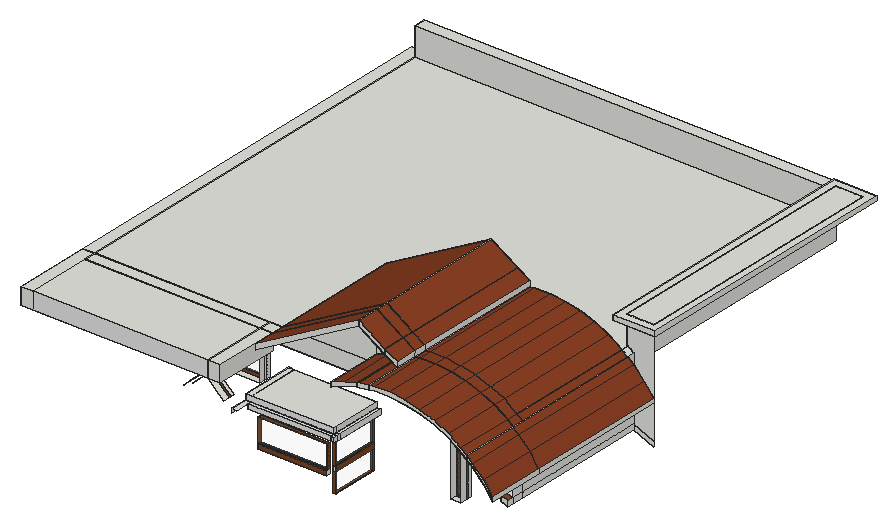
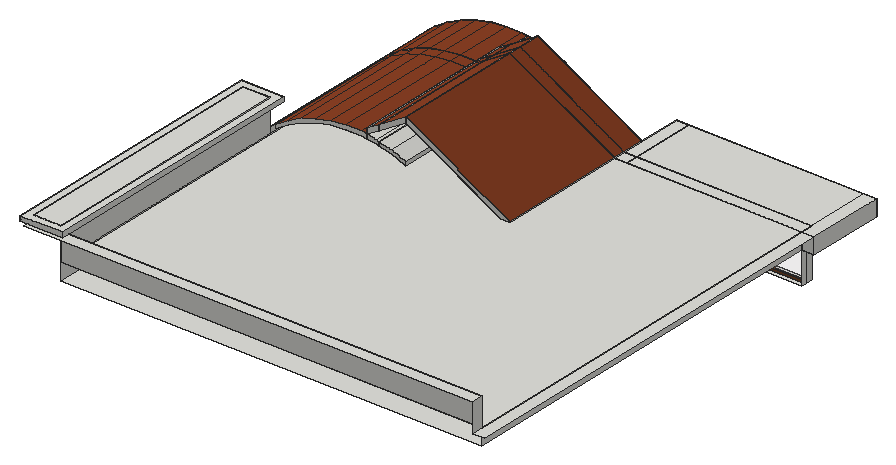
# SketchUp Ruby script. Lengths in inches.
U = 1.inch
M = Sketchup.active_model
def pt(a) = Geom::Point3d.new(a.map { |v| v * U })
def face(e, loops, mat)
  f = e.add_face(loops[0].map { |a| pt(a) })
  loops[1..].each { |l| e.add_face(l.map { |a| pt(a) }).erase! }
  f.material = f.back_material = mat if mat
  f
end
# faces: each face lists its corners as indices into pts; further lists are holes
def faces(e, pts, list, mat = nil) = list.each { |f| face(e, (f[0].is_a?(Array) ? f : [f]).map { |l| l.map { |i| pts[i] } }, mat) }
# xy, xz, yz: faces in a plane at the given z, y or x. An outline is a flat list of corners, or four numbers for a rectangle; further outlines are holes
def ring(l) = l.size == 4 ? [[l[0], l[1]], [l[2], l[1]], [l[2], l[3]], [l[0], l[3]]] : l.each_slice(2).to_a
def flat(e, list, mat, &to3) = list.each { |f| face(e, (f[0].is_a?(Array) ? f : [f]).map { |l| ring(l).map { |u, v| to3.(u, v) } }, mat) }
def xy(e, z, list, mat = nil) = flat(e, list, mat) { |x, y| [x, y, z] }
def xz(e, y, list, mat = nil) = flat(e, list, mat) { |x, z| [x, y, z] }
def yz(e, x, list, mat = nil) = flat(e, list, mat) { |y, z| [x, y, z] }
def lines(e, pts, list) = list.each { |a, b| e.add_line(pt(pts[a]), pt(pts[b])) }
# prism: a flat outline (further loops are holes) pulled along v
def prism(e, loops, v, mat = nil)
  f = face(e, loops, mat); d = Geom::Vector3d.new(v.map { |x| x * U })
  f.pushpull(f.normal.samedirection?(d) ? d.length : -d.length)
end
def box(e, o, s, mat = nil) = prism(e, [[o, [o[0] + s[0], o[1], o[2]], [o[0] + s[0], o[1] + s[1], o[2]], [o[0], o[1] + s[1], o[2]]]], [0, 0, s[2]], mat)
def at(x, y, z, deg = 0) = Geom::Transformation.translation(pt([x, y, z])) * Geom::Transformation.rotation(ORIGIN, Z_AXIS, deg.degrees)
def axes(o, x, y, z) = Geom::Transformation.new([*x, 0, *y, 0, *z, 0, *pt(o).to_a, 1])
def part(name) = M.definitions.add(name)
# library, detail: a bought-in or finely detailed component or shape, given as its bounding box
def library(name, o, s) = part(name).tap { |d| box(d.entities, o, s) }
def detail(e, o, s) = box(e.add_group.entities, o, s)
def put(e, d, t, mat = nil) = e.add_instance(d, t).tap { |i| i.material = mat if mat }
def group(e, t, mat = nil) = e.add_group.tap { |g| g.transformation = t; g.material = mat if mat }.entities
root = M.entities
M.materials.add("Glass Thin Clear 001").color = [243, 240, 240]
M.materials["Glass Thin Clear 001"].alpha = 0.1
M.materials.add("[Color M01]").color = [226, 226, 226]
M.materials.add("[Roofing Tile Spanish]").color = [138, 64, 36]
M.materials.add("[Wood Veneer 01]").color = [120, 70, 37]
xy(root,188.71,[[288.03,166.0625,295.34,170.5625],[288.03,170.5625,295.34,172.4375],[288.03,172.4375,295.34,172.5],[288.03,172.5,295.34,175.0625]])
xy(root,189.01,[[231.27,128.93,233.15,163.51],[233.15,128.93,233.59,163.51]],"[Wood Veneer 01]")
xy(root,189.7,[[289.02,170.5625,294.34,171.125],[289.02,171.125,294.34,172.5]],"[Wood Veneer 01]")
xy(root,200.48,[[177.78,126.375,228.77,127],[177.78,127,228.77,128.9375]],"[Wood Veneer 01]")
xy(root,203.62,[[231.27,128.93,233.15,163.51],[233.15,128.93,233.59,163.51]],"[Wood Veneer 01]")
xy(root,203.86,[[177.78,126.375,228.77,127],[177.78,127,228.77,128.9375]],"[Wood Veneer 01]")
xy(root,207.19,[[231.27,128.93,233.15,163.51],[233.15,128.93,233.59,163.51]],"[Wood Veneer 01]")
xy(root,216.17,[[18.96,166.0625,147.96,170.5625],[18.96,171.875,147.96,175.0625]])
xy(root,216.17,[[18.96,170.5625,147.96,171.5625],[18.96,171.5625,147.96,171.875]],"[Wood Veneer 01]")
xy(root,217.66,[[42.44,170.5625,44.71,171.875],[66.82,170.5625,69.08,171.875],[89.69,170.5625,91.96,171.875],[117,170.5625,119.27,171.875]])
xy(root,217.66,[[20.45,170.5625,42.44,170.875],[44.71,170.5625,66.82,170.875],[69.08,170.5625,89.69,170.875],[91.96,170.5625,117,170.875],[119.27,170.5625,146.47,170.875],
  [20.45,170.875,42.44,171.875],[44.71,170.875,66.82,171.875],[69.08,170.875,89.69,171.875],[91.96,170.875,117,171.875],[119.27,170.875,146.47,171.875]],"[Wood Veneer 01]")
xy(root,221.31,[[177.78,126.375,228.77,127],[177.78,127,228.77,128.9375]],"[Wood Veneer 01]")
xy(root,223.57,[[231.27,128.93,233.15,163.51],[233.15,128.93,233.59,163.51]],"[Wood Veneer 01]")
xy(root,226.125,[[172.96,123.625,233.59,126.375],[233.59,123.625,236.34,126.375],[168.96,126.375,172.96,166.0625],[172.96,126.375,231.27,128.3125],[233.59,126.375,236.34,128.5625],
  [172.96,128.3125,231.27,128.5625],[172.96,128.5625,231.27,128.9375],[233.59,128.5625,236.34,166.0625],[172.96,128.9375,231.27,166.0625],[231.34,128.9375,231.84,166.0625]])
xy(root,226.125,[[231.27,126.375,231.84,128.3125],[231.84,126.375,233.59,128.3125],[231.27,128.3125,231.84,128.5625],[231.84,128.3125,233.59,128.5625],[231.27,128.5625,231.34,128.9375],
  [231.34,128.5625,231.84,128.9375],[231.84,128.5625,233.59,128.9375],[231.27,128.9375,231.34,166.0625],[231.84,128.9375,233.59,166.0625]],"[Wood Veneer 01]")
xy(root,229.5625,[[168.96,113.5625,172.96,126.375],[172.96,123.625,233.59,126.375],[233.59,123.625,236.34,126.375],[168.96,126.375,172.96,166.0625],[172.96,126.375,233.59,128.5625],
  [233.59,126.375,236.34,128.5625],[172.96,128.5625,173.02,166.0625],[173.02,128.5625,233.59,166.0625],[233.59,128.5625,236.34,166.0625]])
xy(root,233.5,[[168.96,126.375,233.59,126.375,233.59,166.0625,173.02,166.0625,173.02,128.5625,172.96,128.5625,172.96,166.0625,168.96,166.0625],[172.96,128.5625,173.02,166.0625]])
xy(root,238.51,[[20.45,170.5625,42.44,170.875],[42.44,170.5625,44.71,171.875],[66.82,170.5625,69.08,171.875],[89.69,170.5625,91.96,171.875],[117,170.5625,119.27,171.875],
  [119.27,170.875,146.47,171.875]])
xy(root,238.51,[[44.71,170.5625,66.82,170.875],[69.08,170.5625,89.69,170.875],[91.96,170.5625,117,170.875],[119.27,170.5625,146.47,170.875],[20.45,170.875,42.44,171.875],
  [44.71,170.875,66.82,171.875],[69.08,170.875,89.69,171.875],[91.96,170.875,117,171.875]],"[Wood Veneer 01]")
xy(root,240,[[9.96,118.0625,18.96,166.0625],[18.96,118.0625,147.96,166.0625],[147.96,118.0625,156.96,166.0625],[9.96,166.0625,18.96,175.0625],[18.96,175.0625,328.85,469.0625]])
xy(root,240,[[18.96,170.5625,147.96,171.5625],[18.96,171.5625,147.96,171.875]],"[Wood Veneer 01]")
xy(root,252,[[9.96,118.0625,18.96,175.0625],[18.96,118.0625,147.96,166.0625],[147.96,118.0625,156.96,166.0625],[18.96,166.0625,147.96,175.0625],[147.96,166.0625,156.96,175.0625],
  [9.96,175.0625,18.96,478.0625],[18.96,175.0625,328.85,469.0625]])
xy(root,258.59,[[289.02,170.5625,294.34,171.125],[289.02,171.125,294.34,172.5]],"[Wood Veneer 01]")
xy(root,259.58,[[288.03,166.0625,295.34,170.5625],[288.03,172.5,295.34,175.0625]])
xy(root,259.58,[[288.03,170.5625,295.34,172.4375],[288.03,172.4375,295.34,172.5]],"[Wood Veneer 01]")
xy(root,259.6875,[[274.03,170.5625,280.57,171.125],[274.03,171.125,280.57,172.5]],"[Wood Veneer 01]")
xy(root,259.97,[[259.4375,170.5625,266.9,171.125],[259.4375,171.125,266.9,172.5]],"[Wood Veneer 01]")
xy(root,260.53,[[244.43,170.5625,251.95,170.8125],[244.43,170.8125,251.95,172.5]],"[Wood Veneer 01]")
xy(root,260.67,[[273.05,166.0625,281.55,170.5625],[273.05,172.5,281.55,175.0625]])
xy(root,260.67,[[273.05,170.5625,281.55,172.4375],[273.05,172.4375,281.55,172.5]],"[Wood Veneer 01]")
xy(root,261.18,[[258.23,166.0625,268.1,170.5625],[258.23,172.5,268.1,175.0625]])
xy(root,261.18,[[258.23,170.5625,268.1,172.4375],[258.23,172.4375,268.1,172.5]],"[Wood Veneer 01]")
xy(root,261.4,[[243.5625,166.0625,252.8125,170.5625],[243.5625,172.5,252.8125,175.0625]])
xy(root,261.4,[[243.5625,170.5625,252.8125,172.125],[243.5625,172.125,252.8125,172.5]],"[Wood Veneer 01]")
xy(root,272.68,[[323.41,271.25,323.41,469.0625,328.85,469.0625,328.85,276.6875,348.92,276.6875,348.92,474.5,354.36,474.5,354.36,271.25],[328.85,276.6875,348.92,469.0625],[18.96,469.0625,323.41,469.0625,323.41,474.5,348.92,474.5,348.92,478.0625,18.96,478.0625],[323.41,469.0625,348.92,474.5]])
xy(root,276.24,[[[323.41,271.25,354.36,474.5],[328.85,276.6875,348.92,469.0625]],[328.85,276.6875,348.92,469.0625]])
xz(root,118.0625,[[9.96,240,18.96,252],[147.96,240,156.96,252]])
xz(root,118.0625,[[18.96,240,147.96,252]],"[Color M01]")
xz(root,123.625,[[233.59,226.125,236.34,229.5625],[353.03,228.22,353.03,231.22,346.26,240.23,338.49,248.37,333.96,252.11,333.96,249.1,338.49,245.37,346.26,237.22],[333.96,249.1,333.96,252.11,329.8,255.54,320.33,261.63,310.2,266.5625,299.57,270.26,288.57,272.68,277.36,273.78,266.11,273.55,261.96,272.98,261.96,269.97,266.11,270.55,277.36,270.78,288.57,269.67,299.57,267.25,310.2,263.55,320.33,258.625,329.8,252.53],[233.59,262,244.0625,266.13,252.96,268.47,252.96,271.47,244.0625,269.14,233.59,265.01],[252.96,268.47,254.95,268.99,261.96,269.97,261.96,272.98,254.95,272,252.96,271.47]])
xz(root,123.625,[[172.96,226.125,233.59,229.5625]],"[Color M01]")
xz(root,126.375,[[168.96,226.125,172.96,229.5625],[172.96,226.125,233.59,229.5625],[233.59,226.125,236.34,229.5625]])
xz(root,126.375,[[168.96,229.5625,233.59,233.5]],"[Color M01]")
xz(root,126.375,[[177.78,200.48,228.77,203.86]],"[Wood Veneer 01]")
xz(root,127,[[177.78,203.86,228.77,221.31]],"Glass Thin Clear 001")
xz(root,128.5625,[[172.96,226.125,233.59,229.5625],[233.59,226.125,236.34,229.5625],[172.96,229.5625,173.02,233.5]])
xz(root,128.93,[[231.27,203.62,233.59,207.19]])
xz(root,128.93,[[231.27,189.01,233.15,203.62],[233.15,189.01,233.59,203.62],[231.27,207.19,233.15,223.57],[233.15,207.19,233.59,223.57]],"[Wood Veneer 01]")
xz(root,128.9375,[[177.78,200.48,228.77,203.86]],"[Wood Veneer 01]")
xz(root,149.75,[[156.96,248,233.59,290.5,233.59,294.5,156.96,252],[261.96,272.98,261.96,276.98,252.96,282.53,252.96,278.53],[252.96,278.53,252.96,282.53,233.59,294.5,233.59,290.5]])
xz(root,161.1875,[[333.96,201.6875,333.96,205.6875,328.85,207.72,328.85,203.72]])
xz(root,163.51,[[231.27,203.62,233.59,207.19]])
xz(root,163.51,[[231.27,189.01,233.15,203.62],[233.15,189.01,233.59,203.62],[231.27,207.19,233.15,223.57],[233.15,207.19,233.59,223.57]],"[Wood Veneer 01]")
xz(root,166.0625,[[168.96,226.125,172.96,229.5625],[172.96,226.125,233.59,229.5625],[233.59,226.125,236.34,229.5625],[353.03,228.22,346.26,237.22,338.49,245.37,333.96,249.1,333.96,252.11,338.49,248.37,346.26,240.23,353.03,231.22],[168.96,229.5625,172.96,233.5],
  [172.96,229.5625,173.02,233.5],[173.02,229.5625,233.59,233.5],[18.96,240,147.96,252],[147.96,240,156.96,252],[156.96,248,156.96,252,233.59,294.5,233.59,290.5],
  [333.96,249.1,329.8,252.53,320.33,258.625,310.2,263.55,299.57,267.25,288.57,269.67,277.36,270.78,266.11,270.55,261.96,269.97,261.96,272.98,266.11,273.55,277.36,273.78,288.57,272.68,299.57,270.26,310.2,266.5625,320.33,261.63,329.8,255.54,333.96,252.11],[233.59,262,233.59,265.01,244.0625,269.14,252.96,271.47,252.96,268.47,244.0625,266.13],[233.59,265.01,244.0625,269.14,252.96,271.47,252.96,278.53,233.59,290.5],[252.96,268.47,252.96,271.47,254.95,272,261.96,272.98,261.96,269.97,254.95,268.99],[252.96,271.47,254.95,272,261.96,272.98,252.96,278.53],
  [261.96,272.98,252.96,278.53,252.96,282.53,261.96,276.98],[252.96,278.53,233.59,290.5,233.59,294.5,252.96,282.53]])
xz(root,170.5625,[[[288.03,188.71,295.34,259.58],[289.02,189.7,294.34,258.59]],[[18.96,216.17,147.96,240],[20.45,217.66,146.47,238.51]],[42.44,217.66,44.71,238.51],[66.82,217.66,69.08,238.51],[89.69,217.66,91.96,238.51],
  [117,217.66,119.27,238.51]],"[Wood Veneer 01]")
xz(root,170.875,[[20.45,217.66,42.44,238.51],[44.71,217.66,66.82,238.51],[69.08,217.66,89.69,238.51],[91.96,217.66,117,238.51],[119.27,217.66,146.47,238.51]],"Glass Thin Clear 001")
xz(root,171.125,[[289.02,189.7,294.34,258.59]],"Glass Thin Clear 001")
xz(root,171.5625,[[18.96,216.17,147.96,240]],"Glass Thin Clear 001")
xz(root,171.875,[[[18.96,216.17,147.96,240],[20.45,217.66,146.47,238.51]],[42.44,217.66,44.71,238.51],[66.82,217.66,69.08,238.51],[89.69,217.66,91.96,238.51],[117,217.66,119.27,238.51]],"[Wood Veneer 01]")
xz(root,172.4375,[[288.03,188.71,295.34,259.58]],"Glass Thin Clear 001")
xz(root,172.5,[[[288.03,188.71,295.34,259.58],[289.02,189.7,294.34,258.59]]],"[Wood Veneer 01]")
xz(root,175.0625,[[333.96,205.6875,333.96,252.11,329.8,255.54,328.85,207.72],[9.96,240,18.96,252],[18.96,240,147.96,252],[147.96,240,243.5625,252],[243.5625,240,252.8125,252],
  [252.8125,240,252.96,252],[252.96,240,258.23,252],[258.23,240,268.1,252],[268.1,240,273.05,252],[273.05,240,281.55,252],
  [281.55,240,288.03,252],[288.03,240,295.34,252],[295.34,240,328.85,252],[156.96,252,233.59,294.5,252.96,282.53,252.96,252,252.8125,252,252.8125,261.4,243.5625,261.4,243.5625,252]])
xz(root,271.25,[[353.03,228.22,346.26,237.22,338.49,245.37,333.96,249.1,333.96,252.11,338.49,248.37,346.26,240.23,353.03,231.22],[156.96,248,156.96,252,233.59,294.5,233.59,290.5],[333.96,249.1,329.8,252.53,320.33,258.625,310.2,263.55,299.57,267.25,288.57,269.67,277.36,270.78,266.11,270.55,261.96,269.97,261.96,272.98,266.11,273.55,277.36,273.78,288.57,272.68,299.57,270.26,310.2,266.5625,320.33,261.63,329.8,255.54,333.96,252.11],[233.59,262,233.59,265.01,244.0625,269.14,252.96,271.47,252.96,268.47,244.0625,266.13],[252.96,268.47,252.96,271.47,254.95,272,261.96,272.98,261.96,269.97,254.95,268.99],
  [323.41,272.68,354.36,276.24],[261.96,272.98,252.96,278.53,252.96,282.53,261.96,276.98],[252.96,278.53,233.59,290.5,233.59,294.5,252.96,282.53]])
xz(root,276.6875,[[348.92,195.73,348.92,199.73,333.96,205.6875,333.96,252.11,329.8,255.54,328.85,207.72,333.96,205.6875,333.96,201.6875],[348.92,199.73,348.92,272.68,328.85,272.68,328.85,207.72,329.8,255.54,333.96,252.11,333.96,205.6875],[333.96,201.6875,333.96,205.6875,328.85,207.72,328.85,203.72],[333.96,205.6875,328.85,207.72,329.8,255.54,333.96,252.11],[328.85,272.68,348.92,276.24]])
xz(root,469.0625,[[18.96,252,328.85,272.68],[328.85,272.68,348.92,276.24]])
xz(root,474.5,[[323.41,272.68,354.36,276.24]])
yz(root,9.96,[[118.0625,240,175.0625,252]])
yz(root,18.96,[[166.0625,216.17,170.5625,240],[171.875,216.17,175.0625,240],[166.0625,240,175.0625,252],[175.0625,240,469.0625,252],[469.0625,252,478.0625,272.68]])
yz(root,18.96,[[170.5625,216.17,171.5625,240],[171.5625,216.17,171.875,240]],"[Wood Veneer 01]")
yz(root,20.45,[[170.5625,217.66,170.875,238.51]])
yz(root,20.45,[[170.875,217.66,171.875,238.51]],"[Wood Veneer 01]")
yz(root,42.44,[[170.5625,217.66,170.875,238.51],[170.875,217.66,171.875,238.51]],"[Wood Veneer 01]")
yz(root,44.71,[[170.5625,217.66,170.875,238.51]])
yz(root,44.71,[[170.875,217.66,171.875,238.51]],"[Wood Veneer 01]")
yz(root,66.82,[[170.5625,217.66,170.875,238.51],[170.875,217.66,171.875,238.51]],"[Wood Veneer 01]")
yz(root,69.08,[[170.5625,217.66,170.875,238.51]])
yz(root,69.08,[[170.875,217.66,171.875,238.51]],"[Wood Veneer 01]")
yz(root,89.69,[[170.5625,217.66,170.875,238.51],[170.875,217.66,171.875,238.51]],"[Wood Veneer 01]")
yz(root,91.96,[[170.5625,217.66,170.875,238.51],[170.875,217.66,171.875,238.51]],"[Wood Veneer 01]")
yz(root,117,[[170.5625,217.66,170.875,238.51],[170.875,217.66,171.875,238.51]],"[Wood Veneer 01]")
yz(root,119.27,[[170.5625,217.66,170.875,238.51],[170.875,217.66,171.875,238.51]])
yz(root,146.47,[[170.5625,217.66,170.875,238.51],[170.875,217.66,171.875,238.51]],"[Wood Veneer 01]")
yz(root,147.96,[[166.0625,216.17,166.0625,252,175.0625,252,175.0625,216.17,171.875,216.17,171.875,240,170.5625,240,170.5625,216.17],[170.5625,216.17,171.5625,240],[171.5625,216.17,171.875,240],[118.0625,240,166.0625,252]])
yz(root,156.96,[[118.0625,240,166.0625,240,166.0625,248,149.75,248,149.75,252,118.0625,252],[149.75,248,166.0625,252],[166.0625,248,271.25,252]])
yz(root,168.96,[[113.91,226.125,113.5625,229.5625,126.375,229.5625,126.375,226.125],[126.375,226.125,166.0625,229.5625],[126.375,229.5625,166.0625,233.5]])
yz(root,172.96,[[123.625,226.125,126.375,229.5625],[126.375,226.125,128.5625,229.5625],[128.5625,226.125,166.0625,229.5625],[128.5625,229.5625,166.0625,233.5]])
yz(root,173.02,[[128.5625,229.5625,166.0625,233.5]])
yz(root,177.78,[[126.375,200.48,128.9375,203.86]])
yz(root,177.78,[[126.375,203.86,127,221.31],[127,203.86,128.9375,221.31]],"[Wood Veneer 01]")
yz(root,228.77,[[126.375,200.48,128.9375,203.86]])
yz(root,228.77,[[126.375,203.86,127,221.31],[127,203.86,128.9375,221.31]],"[Wood Veneer 01]")
yz(root,231.27,[[128.93,203.62,163.51,207.19]],"[Wood Veneer 01]")
yz(root,233.15,[[128.93,189.01,163.51,203.62],[128.93,207.19,163.51,223.57]],"Glass Thin Clear 001")
yz(root,233.59,[[123.625,226.125,126.375,229.5625],[126.375,226.125,128.5625,229.5625],[128.5625,226.125,166.0625,229.5625],[126.375,229.5625,128.5625,233.5],[128.5625,229.5625,166.0625,233.5],
  [123.625,262,166.0625,265.01],[166.0625,262,271.25,265.01],[149.75,290.5,166.0625,294.5],[166.0625,290.5,271.25,294.5]])
yz(root,233.59,[[128.93,189.01,128.9375,203.62],[128.93,203.62,128.9375,207.19],[128.9375,203.62,163.51,207.19],[128.93,207.19,128.9375,223.57]],"[Wood Veneer 01]")
yz(root,236.34,[[123.625,226.125,126.375,229.5625],[126.375,226.125,128.5625,229.5625],[128.5625,226.125,166.0625,229.5625]])
yz(root,252.96,[[123.625,268.47,166.0625,271.47],[166.0625,268.47,175.0625,271.47],[175.0625,268.47,271.25,271.47],[149.75,278.53,166.0625,282.53],[166.0625,278.53,175.0625,282.53],
  [175.0625,278.53,271.25,282.53]])
yz(root,261.96,[[123.625,269.97,166.0625,272.98],[166.0625,269.97,271.25,272.98],[149.75,272.98,166.0625,276.98],[166.0625,272.98,175.0625,276.98],[175.0625,272.98,271.25,276.98]])
yz(root,288.03,[[166.0625,188.71,170.5625,259.58],[172.5,188.71,175.0625,259.58]])
yz(root,288.03,[[170.5625,188.71,172.4375,259.58],[172.4375,188.71,172.5,259.58]],"[Wood Veneer 01]")
yz(root,289.02,[[170.5625,189.7,171.125,258.59],[171.125,189.7,172.5,258.59]],"[Wood Veneer 01]")
yz(root,294.34,[[170.5625,189.7,171.125,258.59],[171.125,189.7,172.5,258.59]],"[Wood Veneer 01]")
yz(root,295.34,[[166.0625,188.71,170.5625,259.58],[172.5,188.71,175.0625,259.58]])
yz(root,295.34,[[170.5625,188.71,172.4375,259.58],[172.4375,188.71,172.5,259.58]],"[Wood Veneer 01]")
yz(root,323.41,[[271.25,272.68,474.5,276.24]])
yz(root,328.85,[[161.1875,203.72,166.0625,207.72],[166.0625,203.72,276.6875,207.72],[175.0625,240,276.6875,252],[276.6875,240,469.0625,252],[276.6875,252,469.0625,272.68],
  [276.6875,272.68,469.0625,276.24]])
yz(root,333.96,[[161.1875,201.6875,166.0625,205.6875],[166.0625,201.6875,175.0625,205.6875],[175.0625,201.6875,276.6875,205.6875],[166.0625,205.6875,175.0625,249.1],[175.0625,205.6875,276.6875,205.6875,276.6875,252.11,271.25,252.11,271.25,249.1,175.0625,249.1],
  [123.625,249.1,166.0625,252.11],[166.0625,249.1,175.0625,252.11],[175.0625,249.1,271.25,252.11]])
yz(root,348.92,[[276.6875,272.68,469.0625,276.24]])
yz(root,353.03,[[123.625,228.22,166.0625,231.22],[166.0625,228.22,271.25,231.22]])
yz(root,354.36,[[271.25,272.68,474.5,276.24]])
p = [[91.87,166.0625,195.01],[91.87,170.5625,195.01],[106.65,170.5625,208.45],[106.65,166.0625,208.45],[121.43,170.5625,195.01],[121.43,166.0625,195.01],
  [106.65,171.875,208.45],[91.87,171.875,195.01],[94.86,170.875,195.01],[106.65,170.875,205.73],[106.65,170.5625,205.73],[94.86,170.5625,195.01],
  [121.43,171.875,195.01],[118.44,170.875,195.01],[118.44,170.5625,195.01],[106.65,172.4375,205.73],[94.86,172.4375,195.01],[118.44,172.4375,195.01],
  [91.87,172.4375,195.01],[106.65,172.4375,208.45],[121.43,172.4375,195.01],[106.65,175.0625,208.45],[91.87,175.0625,195.01],[121.43,175.0625,195.01],
  [328.85,166.0625,203.72],[333.96,166.0625,201.6875],[333.96,161.1875,201.6875],[328.85,161.1875,203.72],[333.96,175.0625,201.6875],[328.85,276.6875,203.72],
  [333.96,276.6875,201.6875],[333.96,166.0625,205.6875],[328.85,166.0625,207.72],[328.85,161.1875,207.72],[333.96,161.1875,205.6875],[333.96,175.0625,205.6875],
  [328.85,175.0625,207.72],[328.85,276.6875,207.72],[333.96,276.6875,205.6875],[329.8,175.0625,255.54],[329.8,271.25,255.54],[329.8,276.6875,255.54],
  [346.26,166.0625,237.22],[353.03,166.0625,228.22],[353.03,123.625,228.22],[346.26,123.625,237.22],[353.03,271.25,228.22],[346.26,271.25,237.22],
  [353.03,166.0625,231.22],[346.26,166.0625,240.23],[346.26,123.625,240.23],[353.03,123.625,231.22],[346.26,271.25,240.23],[353.03,271.25,231.22],
  [338.49,166.0625,245.37],[338.49,123.625,245.37],[338.49,271.25,245.37],[338.49,166.0625,248.37],[338.49,123.625,248.37],[338.49,271.25,248.37],
  [333.96,166.0625,249.1],[333.96,123.625,249.1],[333.96,175.0625,249.1],[333.96,271.25,249.1],[156.96,166.0625,248],[233.59,166.0625,290.5],
  [233.59,149.75,290.5],[156.96,149.75,248],[233.59,271.25,290.5],[156.96,271.25,248],[333.96,166.0625,252.11],[333.96,123.625,252.11],
  [333.96,175.0625,252.11],[333.96,271.25,252.11],[329.8,166.0625,252.53],[329.8,123.625,252.53],[329.8,271.25,252.53],[233.59,166.0625,294.5],
  [156.96,166.0625,252],[156.96,149.75,252],[233.59,149.75,294.5],[233.59,175.0625,294.5],[156.96,175.0625,252],[156.96,271.25,252],
  [233.59,271.25,294.5],[329.8,166.0625,255.54],[329.8,123.625,255.54],[333.96,276.6875,252.11],[320.33,166.0625,258.625],[320.33,123.625,258.625],
  [320.33,271.25,258.625],[320.33,166.0625,261.63],[320.33,123.625,261.63],[320.33,175.0625,261.63],[320.33,271.25,261.63],[310.2,166.0625,263.55],
  [310.2,123.625,263.55],[310.2,271.25,263.55],[310.2,166.0625,266.5625],[310.2,123.625,266.5625],[310.2,175.0625,266.5625],[310.2,271.25,266.5625],
  [233.59,166.0625,262],[244.0625,166.0625,266.13],[244.0625,123.625,266.13],[233.59,123.625,262],[244.0625,271.25,266.13],[233.59,271.25,262],
  [299.57,166.0625,267.25],[299.57,123.625,267.25],[299.57,271.25,267.25],[244.0625,166.0625,269.14],[233.59,166.0625,265.01],[233.59,123.625,265.01],
  [244.0625,123.625,269.14],[233.59,271.25,265.01],[244.0625,271.25,269.14],[252.96,166.0625,268.47],[252.96,123.625,268.47],[252.96,175.0625,268.47],
  [252.96,271.25,268.47],[299.57,166.0625,270.26],[299.57,123.625,270.26],[299.57,175.0625,270.26],[299.57,271.25,270.26],[288.57,166.0625,269.67],
  [288.57,123.625,269.67],[288.57,271.25,269.67],[254.95,166.0625,268.99],[254.95,123.625,268.99],[254.95,271.25,268.99],[261.96,166.0625,269.97],
  [261.96,123.625,269.97],[261.96,271.25,269.97],[252.96,166.0625,271.47],[252.96,123.625,271.47],[252.96,175.0625,271.47],[252.96,271.25,271.47],
  [277.36,166.0625,270.78],[277.36,123.625,270.78],[277.36,271.25,270.78],[266.11,166.0625,270.55],[266.11,123.625,270.55],[266.11,271.25,270.55],
  [288.57,166.0625,272.68],[288.57,123.625,272.68],[288.57,175.0625,272.68],[288.57,271.25,272.68],[254.95,166.0625,272],[254.95,123.625,272],
  [254.95,271.25,272],[261.96,166.0625,272.98],[261.96,123.625,272.98],[261.96,149.75,272.98],[261.96,175.0625,272.98],[261.96,271.25,272.98],
  [277.36,166.0625,273.78],[277.36,123.625,273.78],[277.36,175.0625,273.78],[277.36,271.25,273.78],[266.11,166.0625,273.55],[266.11,123.625,273.55],
  [252.96,166.0625,278.53],[252.96,149.75,278.53],[252.96,175.0625,278.53],[252.96,271.25,278.53],[266.11,175.0625,273.55],[266.11,271.25,273.55],
  [261.96,166.0625,276.98],[252.96,166.0625,282.53],[252.96,149.75,282.53],[261.96,149.75,276.98],[261.96,175.0625,276.98],[252.96,175.0625,282.53],
  [252.96,271.25,282.53],[261.96,271.25,276.98]]
faces(root,p,[[0,1,2,3],[3,2,4,5],[8,9,10,11],[21,19,18,22],[23,20,19,21],[24,25,26,27],[28,25,24,29,30],[31,35,36,32],
  [37,36,35,38],[36,39,40,41,37],[42,43,44,45],[46,43,42,47],[54,42,45,55],[47,42,54,56],[60,54,55,61],[56,54,60,62,63],
  [64,65,66,67],[68,65,64,69],[74,60,61,75],[62,60,74,76,63],[41,40,73,87],[88,74,75,89],[76,74,88,90],[95,88,89,96],
  [90,88,95,97],[102,103,104,105],[106,103,102,107],[108,95,96,109],[97,95,108,110],[115,112,111,116],[103,117,118,104],[119,117,103,106,120],
  [125,108,109,126],[110,108,125,127],[117,128,129,118],[130,128,117,119,120],[128,131,132,129],[133,131,128,130],[116,111,134,136,137],[138,125,126,139],
  [127,125,138,140],[131,141,142,132],[143,141,131,133],[141,138,139,142],[140,138,141,143],[136,134,148,150,137],[150,148,151,154,155],[162,151,153,163],
  [154,151,162,164,165,155],[65,162,163,66],[164,162,65,68,165]])
faces(root,p,[[6,7,1,2],[12,6,2,4],[9,13,14,10],[15,9,8,16],[17,13,9,15],[18,7,6,19],[19,6,12,20]],"[Wood Veneer 01]")
faces(root,p,[[31,32,33,34],[48,49,50,51],[52,49,48,53],[49,57,58,50],[59,57,49,52],[57,70,71,58],[72,70,57,59,73],[77,78,79,80],
  [78,77,81,82],[83,82,81,84],[70,85,86,71],[85,70,72,39],[40,39,72,73],[85,91,92,86],[91,85,39,93],[94,93,39,40],
  [91,98,99,92],[98,91,93,100],[101,100,93,94],[111,112,113,114],[98,121,122,99],[121,98,100,123],[124,123,100,101],[134,111,114,135],
  [121,144,145,122],[144,121,123,146],[147,146,123,124],[148,134,135,149],[151,148,149,152,153],[144,156,157,145],[156,144,146,158],[159,158,146,147],
  [160,151,153,152,161],[151,160,166,154],[155,154,166,167],[156,160,161,157],[160,156,158,166],[167,166,158,159],[168,169,170,171],[169,168,172,173],
  [174,173,172,175],[169,77,80,170],[77,169,173,81],[84,81,173,174]],"[Roofing Tile Spanish]")
